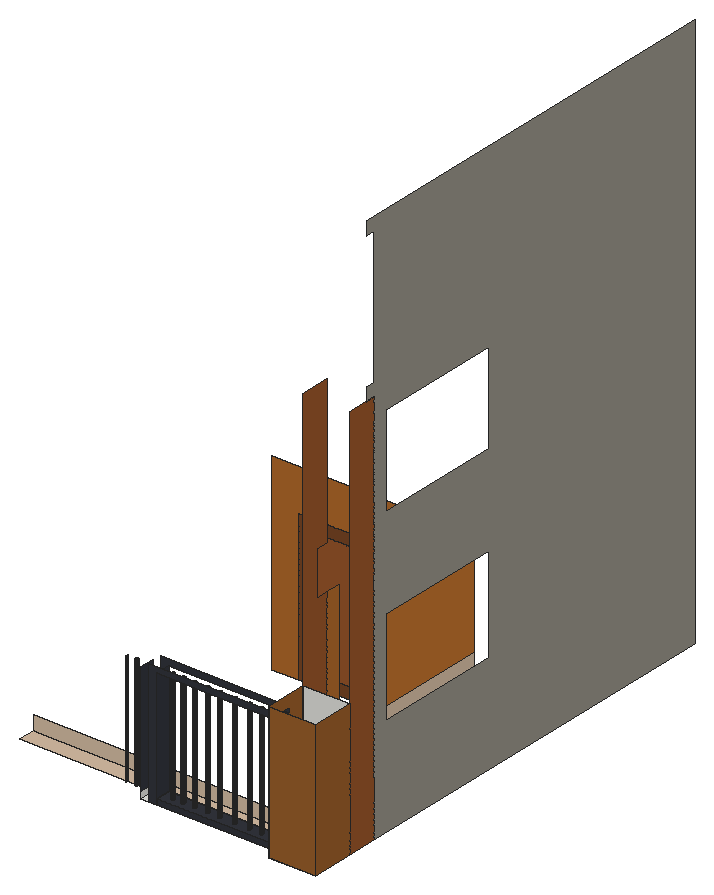
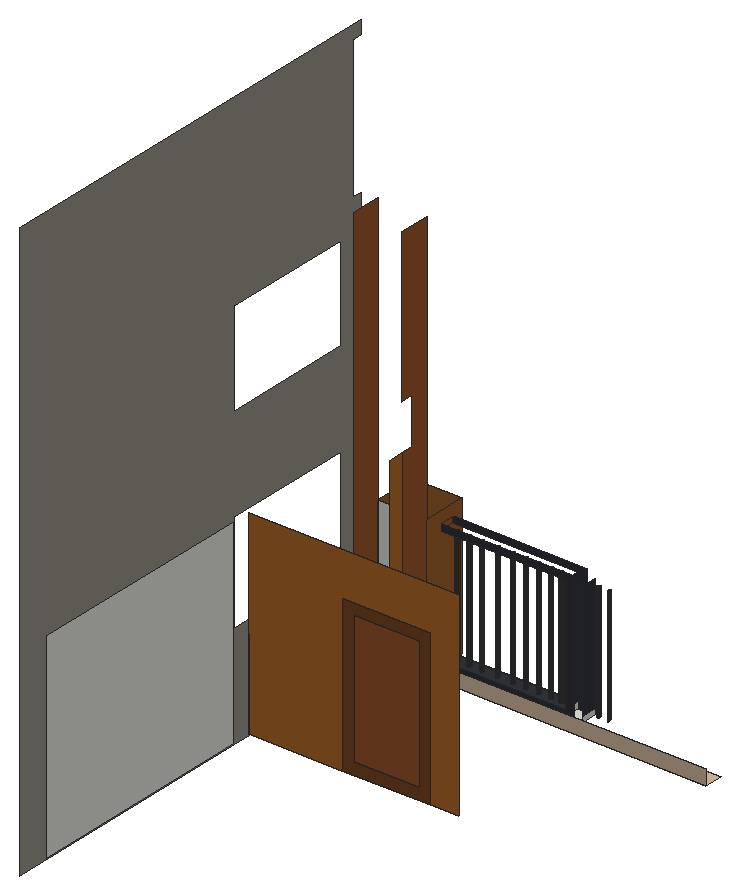
# SketchUp Ruby script. Lengths in inches.
U = 1.inch
M = Sketchup.active_model
def pt(a) = Geom::Point3d.new(a.map { |v| v * U })
def face(e, loops, mat)
  f = e.add_face(loops[0].map { |a| pt(a) })
  loops[1..].each { |l| e.add_face(l.map { |a| pt(a) }).erase! }
  f.material = f.back_material = mat if mat
  f
end
# faces: each face lists its corners as indices into pts; further lists are holes
def faces(e, pts, list, mat = nil) = list.each { |f| face(e, (f[0].is_a?(Array) ? f : [f]).map { |l| l.map { |i| pts[i] } }, mat) }
# xy, xz, yz: faces in a plane at the given z, y or x. An outline is a flat list of corners, or four numbers for a rectangle; further outlines are holes
def ring(l) = l.size == 4 ? [[l[0], l[1]], [l[2], l[1]], [l[2], l[3]], [l[0], l[3]]] : l.each_slice(2).to_a
def flat(e, list, mat, &to3) = list.each { |f| face(e, (f[0].is_a?(Array) ? f : [f]).map { |l| ring(l).map { |u, v| to3.(u, v) } }, mat) }
def xy(e, z, list, mat = nil) = flat(e, list, mat) { |x, y| [x, y, z] }
def xz(e, y, list, mat = nil) = flat(e, list, mat) { |x, z| [x, y, z] }
def yz(e, x, list, mat = nil) = flat(e, list, mat) { |y, z| [x, y, z] }
def lines(e, pts, list) = list.each { |a, b| e.add_line(pt(pts[a]), pt(pts[b])) }
# prism: a flat outline (further loops are holes) pulled along v
def prism(e, loops, v, mat = nil)
  f = face(e, loops, mat); d = Geom::Vector3d.new(v.map { |x| x * U })
  f.pushpull(f.normal.samedirection?(d) ? d.length : -d.length)
end
def box(e, o, s, mat = nil) = prism(e, [[o, [o[0] + s[0], o[1], o[2]], [o[0] + s[0], o[1] + s[1], o[2]], [o[0], o[1] + s[1], o[2]]]], [0, 0, s[2]], mat)
def at(x, y, z, deg = 0) = Geom::Transformation.translation(pt([x, y, z])) * Geom::Transformation.rotation(ORIGIN, Z_AXIS, deg.degrees)
def axes(o, x, y, z) = Geom::Transformation.new([*x, 0, *y, 0, *z, 0, *pt(o).to_a, 1])
def part(name) = M.definitions.add(name)
# library, detail: a bought-in or finely detailed component or shape, given as its bounding box
def library(name, o, s) = part(name).tap { |d| box(d.entities, o, s) }
def detail(e, o, s) = box(e.add_group.entities, o, s)
def put(e, d, t, mat = nil) = e.add_instance(d, t).tap { |i| i.material = mat if mat }
def group(e, t, mat = nil) = e.add_group.tap { |g| g.transformation = t; g.material = mat if mat }.entities
root = M.entities
M.materials.add("[Color M08]").color = [30, 30, 30]
M.materials.add("[Formica Graystone]").color = [149, 146, 135]
M.materials.add("[Formica Laminate Dark]").color = [50, 53, 60]
M.materials.add("[Formica Laminate Light]").color = [213, 189, 164]
M.materials.add("[Wood Bamboo]").color = [177, 105, 43]
M.materials.add("[Wood Cherry Original]").color = [152, 86, 42]
M.materials.add("[Wood Floor Dark]").color = [153, 94, 42]
M.materials.add("[Wood Veneer 01]").color = [120, 70, 37]
xy(root,0,[[504.33,31.06,533.83,57.99],[418.54,37.79,428.66,47.28],[428.66,37.79,504.33,47.28]])
xy(root,0,[[335.09,47.28,504.33,57.99]],"[Formica Laminate Light]")
xy(root,3.5625,[[[428.66,37.79,504.33,47.28],[441.37,41.58,441.11,41.61,440.87,41.71,440.66,41.875,440.51,42.08,440.41,42.32,440.37,42.58,440.41,42.84,440.51,43.08,440.66,43.29,440.87,43.45,441.11,43.55,441.37,43.58,441.63,43.55,441.87,43.45,442.08,43.29,442.24,43.08,442.34,42.84,442.37,42.58,442.34,42.32,442.24,42.08,442.08,41.875,441.87,41.71,441.63,41.61],[448.68,41.58,448.43,41.61,448.18,41.71,447.98,41.875,447.82,42.08,447.72,42.32,447.68,42.58,447.72,42.84,447.82,43.08,447.98,43.29,448.18,43.45,448.43,43.55,448.68,43.58,448.94,43.55,449.18,43.45,449.39,43.29,449.55,43.08,449.65,42.84,449.68,42.58,449.65,42.32,449.55,42.08,449.39,41.875,449.18,41.71,448.94,41.61],[456.56,41.58,456.3,41.61,456.06,41.71,455.85,41.875,455.69,42.08,455.59,42.32,455.56,42.58,455.59,42.84,455.69,43.08,455.85,43.29,456.06,43.45,456.3,43.55,456.56,43.58,456.82,43.55,457.06,43.45,457.27,43.29,457.43,43.08,457.52,42.84,457.56,42.58,457.52,42.32,457.43,42.08,457.27,41.875,457.06,41.71,456.82,41.61],[464.37,41.58,464.11,41.61,463.87,41.71,463.66,41.875,463.51,42.08,463.41,42.32,463.37,42.58,463.41,42.84,463.51,43.08,463.66,43.29,463.87,43.45,464.11,43.55,464.37,43.58,464.63,43.55,464.87,43.45,465.08,43.29,465.24,43.08,465.34,42.84,465.37,42.58,465.34,42.32,465.24,42.08,465.08,41.875,464.87,41.71,464.63,41.61],[473.68,41.58,473.43,41.61,473.18,41.71,472.98,41.875,472.82,42.08,472.72,42.32,472.68,42.58,472.72,42.84,472.82,43.08,472.98,43.29,473.18,43.45,473.43,43.55,473.68,43.58,473.94,43.55,474.18,43.45,474.39,43.29,474.55,43.08,474.65,42.84,474.68,42.58,474.65,42.32,474.55,42.08,474.39,41.875,474.18,41.71,473.94,41.61],[483,41.58,482.74,41.61,482.5,41.71,482.29,41.875,482.13,42.08,482.03,42.32,482,42.58,482.03,42.84,482.13,43.08,482.29,43.29,482.5,43.45,482.74,43.55,483,43.58,483.26,43.55,483.5,43.45,483.7,43.29,483.86,43.08,483.96,42.84,484,42.58,483.96,42.32,483.86,42.08,483.7,41.875,483.5,41.71,483.26,41.61],[490.75,41.58,490.49,41.61,490.25,41.71,490.04,41.875,489.88,42.08,489.78,42.32,489.75,42.58,489.78,42.84,489.88,43.08,490.04,43.29,490.25,43.45,490.49,43.55,490.75,43.58,491.01,43.55,491.25,43.45,491.45,43.29,491.61,43.08,491.71,42.84,491.75,42.58,491.71,42.32,491.61,42.08,491.45,41.875,491.25,41.71,491.01,41.61],[497.93,41.58,497.68,41.61,497.43,41.71,497.23,41.875,497.07,42.08,496.97,42.32,496.93,42.58,496.97,42.84,497.07,43.08,497.23,43.29,497.43,43.45,497.68,43.55,497.93,43.58,498.19,43.55,498.43,43.45,498.64,43.29,498.8,43.08,498.9,42.84,498.93,42.58,498.9,42.32,498.8,42.08,498.64,41.875,498.43,41.71,498.19,41.61],[435,41.58,434.74,41.61,434.5,41.71,434.29,41.875,434.13,42.08,434.03,42.32,434,42.58,434.03,42.84,434.13,43.08,434.29,43.29,434.5,43.45,434.74,43.55,435,43.58,435.26,43.55,435.5,43.45,435.7,43.29,435.86,43.08,435.96,42.84,436,42.58,435.96,42.32,435.86,42.08,435.7,41.875,435.5,41.71,435.26,41.61]]],"[Formica Laminate Dark]")
xz(root,31.06,[[504.33,0,533.83,84.875]],"[Wood Floor Dark]")
xz(root,37.79,[[423.6,0,428.66,0,428.66,74.1,504.33,74.1,504.33,77.6875,423.6,77.6875],[428.66,0,504.33,3.5625]],"[Formica Laminate Dark]")
xz(root,47.28,[[423.6,0,423.6,77.6875,504.33,77.6875,504.33,74.1,428.66,74.1,428.66,0],[428.66,0,504.33,3.5625]],"[Formica Laminate Dark]")
xz(root,57.99,[[504.33,0,533.83,84.875]])
xz(root,57.99,[[335.09,0,504.33,9]],"[Formica Laminate Light]")
xz(root,85.74,[[504.33,9,524.83,62.9375]],"[Formica Graystone]")
xz(root,166.38,[[398.15,9,414.85,9,414.85,102.625,468.53,102.625,468.53,9,524.83,9,524.83,129,398.15,129]],"[Wood Bamboo]")
xz(root,166.38,[[422.21,16.36,461.17,95.26]],"[Wood Cherry Original]")
xz(root,166.38,[[[414.85,9,468.53,102.625],[422.21,16.36,461.17,95.26]]],"[Wood Veneer 01]")
yz(root,418.54,[[37.79,0,47.28,3.5625]])
yz(root,418.54,[[37.79,3.5625,47.28,74.1]],"[Formica Laminate Dark]")
yz(root,428.66,[[37.79,0,47.28,3.5625]])
yz(root,428.66,[[37.79,3.5625,47.28,74.1]],"[Formica Laminate Dark]")
yz(root,504.33,[[37.79,0,47.28,3.5625]])
yz(root,504.33,[[76.74,9,85.74,129]],"[Wood Bamboo]")
yz(root,504.33,[[57.99,9,57.99,249,76.74,249,76.74,157,68.99,157,68.99,129,76.74,129,76.74,9]],"[Wood Cherry Original]")
yz(root,504.33,[[[31.06,0,31.06,84.875,57.99,84.875,57.99,0,47.28,0,47.28,3.5625,37.79,3.5625,37.79,0],[37.79,74.1,47.28,77.6875]]],"[Wood Floor Dark]")
yz(root,524.83,[[178.72,9,319.17,129]])
yz(root,524.83,[[85.74,9,166.38,62.9375]],"[Formica Laminate Light]")
yz(root,533.83,[[[76.74,0,328.17,0,328.17,350.875,70.93,350.875,70.93,342.48,76.74,342.48,76.74,257.39,70.93,257.39,70.93,249,76.74,249],[85.74,62.9375,166.38,123.3125],[85.74,180.5625,166.38,237.86]]],"[Formica Graystone]")
yz(root,533.83,[[57.99,0,76.74,249]],"[Wood Cherry Original]")
yz(root,533.83,[[31.06,0,57.99,84.875]],"[Wood Floor Dark]")
p = [[412.05,41.61,74.1],[411.81,41.71,74.1],[411.81,41.71,3.5625],[412.05,41.61,3.5625],[412.31,41.58,74.1],[412.31,41.58,3.5625],
  [412.57,41.61,74.1],[412.57,41.61,3.5625],[412.81,41.71,74.1],[412.81,41.71,3.5625],[434.74,41.61,74.1],[434.5,41.71,74.1],
  [434.5,41.71,3.5625],[434.74,41.61,3.5625],[435,41.58,74.1],[435,41.58,3.5625],[435.26,41.61,74.1],[435.26,41.61,3.5625],
  [435.5,41.71,74.1],[435.5,41.71,3.5625],[441.11,41.61,74.1],[440.87,41.71,74.1],[440.87,41.71,3.5625],[441.11,41.61,3.5625],
  [441.37,41.58,74.1],[441.37,41.58,3.5625],[441.63,41.61,74.1],[441.63,41.61,3.5625],[441.87,41.71,74.1],[441.87,41.71,3.5625],
  [448.43,41.61,73.98],[448.18,41.71,73.98],[448.18,41.71,3.5625],[448.43,41.61,3.5625],[448.68,41.58,73.98],[448.68,41.58,3.5625],
  [448.94,41.61,73.98],[448.94,41.61,3.5625],[449.18,41.71,73.98],[449.18,41.71,3.5625],[456.3,41.61,74.1],[456.06,41.71,74.1],
  [456.06,41.71,3.5625],[456.3,41.61,3.5625],[456.56,41.58,74.1],[456.56,41.58,3.5625],[456.82,41.61,74.1],[456.82,41.61,3.5625],
  [457.06,41.71,74.1],[457.06,41.71,3.5625],[464.11,41.61,74.1],[463.87,41.71,74.1],[463.87,41.71,3.5625],[464.11,41.61,3.5625],
  [464.37,41.58,74.1],[464.37,41.58,3.5625],[464.63,41.61,74.1],[464.63,41.61,3.5625],[464.87,41.71,74.1],[464.87,41.71,3.5625],
  [473.43,41.61,74.1],[473.18,41.71,74.1],[473.18,41.71,3.5625],[473.43,41.61,3.5625],[473.68,41.58,74.1],[473.68,41.58,3.5625],
  [473.94,41.61,74.1],[473.94,41.61,3.5625],[474.18,41.71,74.1],[474.18,41.71,3.5625],[482.74,41.61,74.1],[482.5,41.71,74.1],
  [482.5,41.71,3.5625],[482.74,41.61,3.5625],[483,41.58,74.1],[483,41.58,3.5625],[483.26,41.61,74.1],[483.26,41.61,3.5625],
  [483.5,41.71,74.1],[483.5,41.71,3.5625],[490.49,41.61,74.1],[490.25,41.71,74.1],[490.25,41.71,3.5625],[490.49,41.61,3.5625],
  [490.75,41.58,74.1],[490.75,41.58,3.5625],[491.01,41.61,74.1],[491.01,41.61,3.5625],[491.25,41.71,74.1],[491.25,41.71,3.5625],
  [497.68,41.61,74.1],[497.43,41.71,74.1],[497.43,41.71,3.5625],[497.68,41.61,3.5625],[497.93,41.58,74.1],[497.93,41.58,3.5625],
  [498.19,41.61,74.1],[498.19,41.61,3.5625],[498.43,41.71,74.1],[498.43,41.71,3.5625],[406.27,41.875,74.1],[406.06,41.71,74.1],
  [406.06,41.71,3.5625],[406.27,41.875,3.5625],[411.6,41.875,74.1],[411.6,41.875,3.5625],[413.02,41.875,74.1],[413.02,41.875,3.5625],
  [434.29,41.875,74.1],[434.29,41.875,3.5625],[435.7,41.875,74.1],[435.7,41.875,3.5625],[440.66,41.875,74.1],[440.66,41.875,3.5625],
  [442.08,41.875,74.1],[442.08,41.875,3.5625],[447.98,41.875,73.98],[447.98,41.875,3.5625],[449.39,41.875,73.98],[449.39,41.875,3.5625],
  [455.85,41.875,74.1],[455.85,41.875,3.5625],[457.27,41.875,74.1],[457.27,41.875,3.5625],[463.66,41.875,74.1],[463.66,41.875,3.5625],
  [465.08,41.875,74.1],[465.08,41.875,3.5625],[472.98,41.875,74.1],[472.98,41.875,3.5625],[474.39,41.875,74.1],[474.39,41.875,3.5625],
  [482.29,41.875,74.1],[482.29,41.875,3.5625],[483.7,41.875,74.1],[483.7,41.875,3.5625],[490.04,41.875,74.1],[490.04,41.875,3.5625],
  [491.45,41.875,74.1],[491.45,41.875,3.5625],[497.23,41.875,74.1],[497.23,41.875,3.5625],[498.64,41.875,74.1],[498.64,41.875,3.5625],
  [406.43,42.08,74.1],[406.43,42.08,3.5625],[411.44,42.08,74.1],[411.44,42.08,3.5625],[413.18,42.08,74.1],[413.18,42.08,3.5625],
  [434.13,42.08,74.1],[434.13,42.08,3.5625],[435.86,42.08,74.1],[435.86,42.08,3.5625],[440.51,42.08,74.1],[440.51,42.08,3.5625],
  [442.24,42.08,74.1],[442.24,42.08,3.5625],[447.82,42.08,73.98],[447.82,42.08,3.5625],[449.55,42.08,73.98],[449.55,42.08,3.5625],
  [455.69,42.08,74.1],[455.69,42.08,3.5625],[457.43,42.08,74.1],[457.43,42.08,3.5625],[463.51,42.08,74.1],[463.51,42.08,3.5625],
  [465.24,42.08,74.1],[465.24,42.08,3.5625],[472.82,42.08,74.1],[472.82,42.08,3.5625],[474.55,42.08,74.1],[474.55,42.08,3.5625],
  [482.13,42.08,74.1],[482.13,42.08,3.5625],[483.86,42.08,74.1],[483.86,42.08,3.5625],[489.88,42.08,74.1],[489.88,42.08,3.5625],
  [491.61,42.08,74.1],[491.61,42.08,3.5625],[497.07,42.08,74.1],[497.07,42.08,3.5625],[498.8,42.08,74.1],[498.8,42.08,3.5625],
  [406.52,42.32,74.1],[406.52,42.32,3.5625],[411.34,42.32,74.1],[411.34,42.32,3.5625],[413.27,42.32,74.1],[413.27,42.32,3.5625],
  [434.03,42.32,74.1],[434.03,42.32,3.5625],[435.96,42.32,74.1],[435.96,42.32,3.5625],[440.41,42.32,74.1],[440.41,42.32,3.5625],
  [442.34,42.32,74.1],[442.34,42.32,3.5625],[447.72,42.32,73.98],[447.72,42.32,3.5625],[449.65,42.32,73.98],[449.65,42.32,3.5625],
  [455.59,42.32,74.1],[455.59,42.32,3.5625],[457.52,42.32,74.1],[457.52,42.32,3.5625],[463.41,42.32,74.1],[463.41,42.32,3.5625],
  [465.34,42.32,74.1],[465.34,42.32,3.5625],[472.72,42.32,74.1],[472.72,42.32,3.5625],[474.65,42.32,74.1],[474.65,42.32,3.5625],
  [482.03,42.32,74.1],[482.03,42.32,3.5625],[483.96,42.32,74.1],[483.96,42.32,3.5625],[489.78,42.32,74.1],[489.78,42.32,3.5625],
  [491.71,42.32,74.1],[491.71,42.32,3.5625],[496.97,42.32,74.1],[496.97,42.32,3.5625],[498.9,42.32,74.1],[498.9,42.32,3.5625],
  [406.56,42.58,74.1],[406.56,42.58,3.5625],[411.31,42.58,74.1],[411.31,42.58,3.5625],[413.31,42.58,74.1],[413.31,42.58,3.5625],
  [434,42.58,74.1],[434,42.58,3.5625],[436,42.58,74.1],[436,42.58,3.5625],[440.37,42.58,74.1],[440.37,42.58,3.5625],
  [442.37,42.58,74.1],[442.37,42.58,3.5625],[447.68,42.58,73.98],[447.68,42.58,3.5625],[449.68,42.58,73.98],[449.68,42.58,3.5625],
  [455.56,42.58,74.1],[455.56,42.58,3.5625],[457.56,42.58,74.1],[457.56,42.58,3.5625],[463.37,42.58,74.1],[463.37,42.58,3.5625],
  [465.37,42.58,74.1],[465.37,42.58,3.5625],[472.68,42.58,74.1],[472.68,42.58,3.5625],[474.68,42.58,74.1],[474.68,42.58,3.5625],
  [482,42.58,74.1],[482,42.58,3.5625],[484,42.58,74.1],[484,42.58,3.5625],[489.75,42.58,74.1],[489.75,42.58,3.5625],
  [491.75,42.58,74.1],[491.75,42.58,3.5625],[496.93,42.58,74.1],[496.93,42.58,3.5625],[498.93,42.58,74.1],[498.93,42.58,3.5625],
  [406.52,42.84,74.1],[406.52,42.84,3.5625],[411.34,42.84,74.1],[411.34,42.84,3.5625],[413.27,42.84,74.1],[413.27,42.84,3.5625],
  [434.03,42.84,74.1],[434.03,42.84,3.5625],[435.96,42.84,74.1],[435.96,42.84,3.5625],[440.41,42.84,74.1],[440.41,42.84,3.5625],
  [442.34,42.84,74.1],[442.34,42.84,3.5625],[447.72,42.84,73.98],[447.72,42.84,3.5625],[449.65,42.84,73.98],[449.65,42.84,3.5625],
  [455.59,42.84,74.1],[455.59,42.84,3.5625],[457.52,42.84,74.1],[457.52,42.84,3.5625],[463.41,42.84,74.1],[463.41,42.84,3.5625],
  [465.34,42.84,74.1],[465.34,42.84,3.5625],[472.72,42.84,74.1],[472.72,42.84,3.5625],[474.65,42.84,74.1],[474.65,42.84,3.5625],
  [482.03,42.84,74.1],[482.03,42.84,3.5625],[483.96,42.84,74.1],[483.96,42.84,3.5625],[489.78,42.84,74.1],[489.78,42.84,3.5625],
  [491.71,42.84,74.1],[491.71,42.84,3.5625],[496.97,42.84,74.1],[496.97,42.84,3.5625],[498.9,42.84,74.1],[498.9,42.84,3.5625],
  [406.43,43.08,74.1],[406.43,43.08,3.5625],[411.44,43.08,74.1],[411.44,43.08,3.5625],[413.18,43.08,74.1],[413.18,43.08,3.5625],
  [434.13,43.08,74.1],[434.13,43.08,3.5625],[435.86,43.08,74.1],[435.86,43.08,3.5625],[440.51,43.08,74.1],[440.51,43.08,3.5625],
  [442.24,43.08,74.1],[442.24,43.08,3.5625],[447.82,43.08,73.98],[447.82,43.08,3.5625],[449.55,43.08,73.98],[449.55,43.08,3.5625],
  [455.69,43.08,74.1],[455.69,43.08,3.5625],[457.43,43.08,74.1],[457.43,43.08,3.5625],[463.51,43.08,74.1],[463.51,43.08,3.5625],
  [465.24,43.08,74.1],[465.24,43.08,3.5625],[472.82,43.08,74.1],[472.82,43.08,3.5625],[474.55,43.08,74.1],[474.55,43.08,3.5625],
  [482.13,43.08,74.1],[482.13,43.08,3.5625],[483.86,43.08,74.1],[483.86,43.08,3.5625],[489.88,43.08,74.1],[489.88,43.08,3.5625],
  [491.61,43.08,74.1],[491.61,43.08,3.5625],[497.07,43.08,74.1],[497.07,43.08,3.5625],[498.8,43.08,74.1],[498.8,43.08,3.5625],
  [406.27,43.29,74.1],[406.27,43.29,3.5625],[411.6,43.29,74.1],[411.6,43.29,3.5625],[413.02,43.29,74.1],[413.02,43.29,3.5625],
  [434.29,43.29,74.1],[434.29,43.29,3.5625],[435.7,43.29,74.1],[435.7,43.29,3.5625],[440.66,43.29,74.1],[440.66,43.29,3.5625],
  [442.08,43.29,74.1],[442.08,43.29,3.5625],[447.98,43.29,73.98],[447.98,43.29,3.5625],[449.39,43.29,73.98],[449.39,43.29,3.5625],
  [455.85,43.29,74.1],[455.85,43.29,3.5625],[457.27,43.29,74.1],[457.27,43.29,3.5625],[463.66,43.29,74.1],[463.66,43.29,3.5625],
  [465.08,43.29,74.1],[465.08,43.29,3.5625],[472.98,43.29,74.1],[472.98,43.29,3.5625],[474.39,43.29,74.1],[474.39,43.29,3.5625],
  [482.29,43.29,74.1],[482.29,43.29,3.5625],[483.7,43.29,74.1],[483.7,43.29,3.5625],[490.04,43.29,74.1],[490.04,43.29,3.5625],
  [491.45,43.29,74.1],[491.45,43.29,3.5625],[497.23,43.29,74.1],[497.23,43.29,3.5625],[498.64,43.29,74.1],[498.64,43.29,3.5625],
  [406.06,43.45,74.1],[406.06,43.45,3.5625],[411.81,43.45,74.1],[411.81,43.45,3.5625],[412.81,43.45,74.1],[412.81,43.45,3.5625],
  [434.5,43.45,74.1],[434.5,43.45,3.5625],[435.5,43.45,74.1],[435.5,43.45,3.5625],[440.87,43.45,74.1],[440.87,43.45,3.5625],
  [441.87,43.45,74.1],[441.87,43.45,3.5625],[448.18,43.45,73.98],[448.18,43.45,3.5625],[449.18,43.45,73.98],[449.18,43.45,3.5625],
  [456.06,43.45,74.1],[456.06,43.45,3.5625],[457.06,43.45,74.1],[457.06,43.45,3.5625],[463.87,43.45,74.1],[463.87,43.45,3.5625],
  [464.87,43.45,74.1],[464.87,43.45,3.5625],[473.18,43.45,74.1],[473.18,43.45,3.5625],[474.18,43.45,74.1],[474.18,43.45,3.5625],
  [482.5,43.45,74.1],[482.5,43.45,3.5625],[483.5,43.45,74.1],[483.5,43.45,3.5625],[490.25,43.45,74.1],[490.25,43.45,3.5625],
  [491.25,43.45,74.1],[491.25,43.45,3.5625],[497.43,43.45,74.1],[497.43,43.45,3.5625],[498.43,43.45,74.1],[498.43,43.45,3.5625],
  [405.82,43.55,74.1],[405.82,43.55,3.5625],[412.05,43.55,74.1],[412.05,43.55,3.5625],[412.57,43.55,74.1],[412.57,43.55,3.5625],
  [434.74,43.55,74.1],[434.74,43.55,3.5625],[435.26,43.55,74.1],[435.26,43.55,3.5625],[441.11,43.55,74.1],[441.11,43.55,3.5625],
  [441.63,43.55,74.1],[441.63,43.55,3.5625],[448.43,43.55,73.98],[448.43,43.55,3.5625],[448.94,43.55,73.98],[448.94,43.55,3.5625],
  [456.3,43.55,74.1],[456.3,43.55,3.5625],[456.82,43.55,74.1],[456.82,43.55,3.5625],[464.11,43.55,74.1],[464.11,43.55,3.5625],
  [464.63,43.55,74.1],[464.63,43.55,3.5625],[473.43,43.55,74.1],[473.43,43.55,3.5625],[473.94,43.55,74.1],[473.94,43.55,3.5625],
  [482.74,43.55,74.1],[482.74,43.55,3.5625],[483.26,43.55,74.1],[483.26,43.55,3.5625],[490.49,43.55,74.1],[490.49,43.55,3.5625],
  [491.01,43.55,74.1],[491.01,43.55,3.5625],[497.68,43.55,74.1],[497.68,43.55,3.5625],[498.19,43.55,74.1],[498.19,43.55,3.5625],
  [412.31,43.58,74.1],[412.31,43.58,3.5625],[435,43.58,74.1],[435,43.58,3.5625],[441.37,43.58,74.1],[441.37,43.58,3.5625],
  [448.68,43.58,73.98],[448.68,43.58,3.5625],[456.56,43.58,74.1],[456.56,43.58,3.5625],[464.37,43.58,74.1],[464.37,43.58,3.5625],
  [473.68,43.58,74.1],[473.68,43.58,3.5625],[483,43.58,74.1],[483,43.58,3.5625],[490.75,43.58,74.1],[490.75,43.58,3.5625],
  [497.93,43.58,74.1],[497.93,43.58,3.5625]]
faces(root,p,[[0,1,2,3],[4,0,3,5],[6,4,5,7],[8,6,7,9],[10,11,12,13],[14,10,13,15],[16,14,15,17],[18,16,17,19],
  [20,21,22,23],[24,20,23,25],[26,24,25,27],[28,26,27,29],[30,31,32,33],[34,30,33,35],[36,34,35,37],[38,36,37,39],
  [40,41,42,43],[44,40,43,45],[46,44,45,47],[48,46,47,49],[50,51,52,53],[54,50,53,55],[56,54,55,57],[58,56,57,59],
  [60,61,62,63],[64,60,63,65],[66,64,65,67],[68,66,67,69],[70,71,72,73],[74,70,73,75],[76,74,75,77],[78,76,77,79],
  [80,81,82,83],[84,80,83,85],[86,84,85,87],[88,86,87,89],[90,91,92,93],[94,90,93,95],[96,94,95,97],[98,96,97,99],
  [100,101,102,103],[1,104,105,2],[106,8,9,107],[11,108,109,12],[110,18,19,111],[21,112,113,22],[114,28,29,115],[31,116,117,32],
  [118,38,39,119],[41,120,121,42],[122,48,49,123],[51,124,125,52],[126,58,59,127],[61,128,129,62],[130,68,69,131],[71,132,133,72],
  [134,78,79,135],[81,136,137,82],[138,88,89,139],[91,140,141,92],[142,98,99,143],[144,100,103,145],[104,146,147,105],[148,106,107,149],
  [108,150,151,109],[152,110,111,153],[112,154,155,113],[156,114,115,157],[116,158,159,117],[160,118,119,161],[120,162,163,121],[164,122,123,165],
  [124,166,167,125],[168,126,127,169],[128,170,171,129],[172,130,131,173],[132,174,175,133],[176,134,135,177],[136,178,179,137],[180,138,139,181],
  [140,182,183,141],[184,142,143,185],[186,144,145,187],[146,188,189,147],[190,148,149,191],[150,192,193,151],[194,152,153,195],[154,196,197,155],
  [198,156,157,199],[158,200,201,159],[202,160,161,203],[162,204,205,163],[206,164,165,207],[166,208,209,167],[210,168,169,211],[170,212,213,171],
  [214,172,173,215],[174,216,217,175],[218,176,177,219],[178,220,221,179],[222,180,181,223],[182,224,225,183],[226,184,185,227],[228,186,187,229],
  [188,230,231,189],[232,190,191,233],[192,234,235,193],[236,194,195,237],[196,238,239,197],[240,198,199,241],[200,242,243,201],[244,202,203,245],
  [204,246,247,205],[248,206,207,249],[208,250,251,209],[252,210,211,253],[212,254,255,213],[256,214,215,257],[216,258,259,217],[260,218,219,261],
  [220,262,263,221],[264,222,223,265],[224,266,267,225],[268,226,227,269],[270,228,229,271],[230,272,273,231],[274,232,233,275],[234,276,277,235],
  [278,236,237,279],[238,280,281,239],[282,240,241,283],[242,284,285,243],[286,244,245,287],[246,288,289,247],[290,248,249,291],[250,292,293,251],
  [294,252,253,295],[254,296,297,255],[298,256,257,299],[258,300,301,259],[302,260,261,303],[262,304,305,263],[306,264,265,307],[266,308,309,267],
  [310,268,269,311],[312,270,271,313],[272,314,315,273],[316,274,275,317],[276,318,319,277],[320,278,279,321],[280,322,323,281],[324,282,283,325],
  [284,326,327,285],[328,286,287,329],[288,330,331,289],[332,290,291,333],[292,334,335,293],[336,294,295,337],[296,338,339,297],[340,298,299,341],
  [300,342,343,301],[344,302,303,345],[304,346,347,305],[348,306,307,349],[308,350,351,309],[352,310,311,353],[354,312,313,355],[314,356,357,315],
  [358,316,317,359],[318,360,361,319],[362,320,321,363],[322,364,365,323],[366,324,325,367],[326,368,369,327],[370,328,329,371],[330,372,373,331],
  [374,332,333,375],[334,376,377,335],[378,336,337,379],[338,380,381,339],[382,340,341,383],[342,384,385,343],[386,344,345,387],[346,388,389,347],
  [390,348,349,391],[350,392,393,351],[394,352,353,395],[396,354,355,397],[356,398,399,357],[400,358,359,401],[360,402,403,361],[404,362,363,405],
  [364,406,407,365],[408,366,367,409],[368,410,411,369],[412,370,371,413],[372,414,415,373],[416,374,375,417],[376,418,419,377],[420,378,379,421],
  [380,422,423,381],[424,382,383,425],[384,426,427,385],[428,386,387,429],[388,430,431,389],[432,390,391,433],[392,434,435,393],[436,394,395,437],
  [438,396,397,439],[398,440,441,399],[442,400,401,443],[402,444,445,403],[446,404,405,447],[406,448,449,407],[450,408,409,451],[410,452,453,411],
  [454,412,413,455],[414,456,457,415],[458,416,417,459],[418,460,461,419],[462,420,421,463],[422,464,465,423],[466,424,425,467],[426,468,469,427],
  [470,428,429,471],[430,472,473,431],[474,432,433,475],[434,476,477,435],[478,436,437,479],[440,480,481,441],[480,442,443,481],[444,482,483,445],
  [482,446,447,483],[448,484,485,449],[484,450,451,485],[452,486,487,453],[486,454,455,487],[456,488,489,457],[488,458,459,489],[460,490,491,461],
  [490,462,463,491],[464,492,493,465],[492,466,467,493],[468,494,495,469],[494,470,471,495],[472,496,497,473],[496,474,475,497],[476,498,499,477],
  [498,478,479,499]],"[Color M08]")
